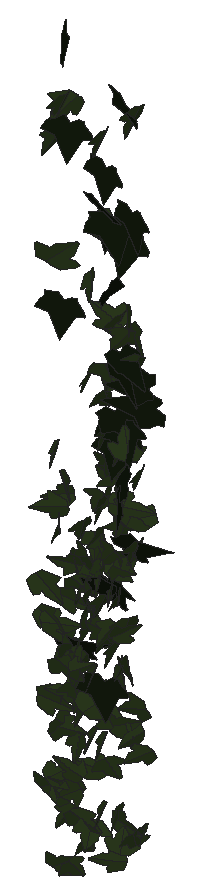
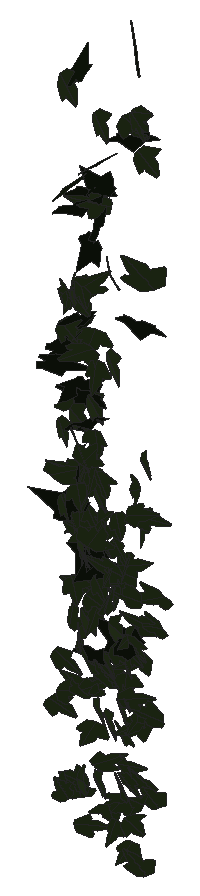
# SketchUp Ruby script. Lengths in inches.
U = 1.inch
M = Sketchup.active_model
def pt(a) = Geom::Point3d.new(a.map { |v| v * U })
def face(e, loops, mat)
  f = e.add_face(loops[0].map { |a| pt(a) })
  loops[1..].each { |l| e.add_face(l.map { |a| pt(a) }).erase! }
  f.material = f.back_material = mat if mat
  f
end
# faces: each face lists its corners as indices into pts; further lists are holes
def faces(e, pts, list, mat = nil) = list.each { |f| face(e, (f[0].is_a?(Array) ? f : [f]).map { |l| l.map { |i| pts[i] } }, mat) }
# xy, xz, yz: faces in a plane at the given z, y or x. An outline is a flat list of corners, or four numbers for a rectangle; further outlines are holes
def ring(l) = l.size == 4 ? [[l[0], l[1]], [l[2], l[1]], [l[2], l[3]], [l[0], l[3]]] : l.each_slice(2).to_a
def flat(e, list, mat, &to3) = list.each { |f| face(e, (f[0].is_a?(Array) ? f : [f]).map { |l| ring(l).map { |u, v| to3.(u, v) } }, mat) }
def xy(e, z, list, mat = nil) = flat(e, list, mat) { |x, y| [x, y, z] }
def xz(e, y, list, mat = nil) = flat(e, list, mat) { |x, z| [x, y, z] }
def yz(e, x, list, mat = nil) = flat(e, list, mat) { |y, z| [x, y, z] }
def lines(e, pts, list) = list.each { |a, b| e.add_line(pt(pts[a]), pt(pts[b])) }
# prism: a flat outline (further loops are holes) pulled along v
def prism(e, loops, v, mat = nil)
  f = face(e, loops, mat); d = Geom::Vector3d.new(v.map { |x| x * U })
  f.pushpull(f.normal.samedirection?(d) ? d.length : -d.length)
end
def box(e, o, s, mat = nil) = prism(e, [[o, [o[0] + s[0], o[1], o[2]], [o[0] + s[0], o[1] + s[1], o[2]], [o[0], o[1] + s[1], o[2]]]], [0, 0, s[2]], mat)
def at(x, y, z, deg = 0) = Geom::Transformation.translation(pt([x, y, z])) * Geom::Transformation.rotation(ORIGIN, Z_AXIS, deg.degrees)
def axes(o, x, y, z) = Geom::Transformation.new([*x, 0, *y, 0, *z, 0, *pt(o).to_a, 1])
def part(name) = M.definitions.add(name)
# library, detail: a bought-in or finely detailed component or shape, given as its bounding box
def library(name, o, s) = part(name).tap { |d| box(d.entities, o, s) }
def detail(e, o, s) = box(e.add_group.entities, o, s)
def put(e, d, t, mat = nil) = e.add_instance(d, t).tap { |i| i.material = mat if mat }
def group(e, t, mat = nil) = e.add_group.tap { |g| g.transformation = t; g.material = mat if mat }.entities
root = M.entities
M.materials.add("1026 AP 7946 SUNNY SIDE UP").color = [254, 231, 186]
M.materials.add("efeu1").color = [18, 25, 13]
M.materials.add("efeu2").color = [43, 57, 29]
c1 = part("ivyleaf_10")
p = [[0,0.5,-0.03],[-0.0625,2.02,-0.43],[-0.19,2.01,-0.46],[-0.54,1.05,-0.29],[-0.52,0.625,-0.18],[-0.83,0.76,-0.28],
  [-1.16,0.64,-0.33],[-1.15,0.33,-0.24],[-0.77,-0.39,0.02],[-0.3,-0.51,0.16],[0.04,-0.48,0.23],[-0.02,2.01,-0.4375],
  [-0.06,2.01,-0.43],[0.04,-0.49,0.23],[0.67,-0.49,0.14],[1.38,0.36,-0.2],[1.375,0.51,-0.24],[0.81,0.65,-0.19],
  [0.62,0.59,-0.15],[0.6,1.09,-0.28],[0.5,1.23,-0.31]]
faces(c1.entities,p,[[0,1,2,3,4,5,6,7,8,9,10],[11,12,0,13,14,15,16,17,18,19,20]],"efeu2")
c2 = part("ivyleaf_9")
p = [[1.54,2.16,1.25],[1.36,2.04,1.19],[-0.21,0.99,0.68],[-0.71,1.11,0.82],[-0.85,0.86,0.67],[-0.8,0.17,0.21],
  [-0.9,-0.01,0.1],[-0.67,-0.16,-0.02],[-0.08,-0.08,-0.05],[-0.03,-0.6,-0.4],[0.65,-0.88,-0.66],[0.83,-0.6,-0.49],
  [1.29,-0.42,-0.43],[1.8125,-0.07,-0.26],[1.21,0.44,0.15]]
faces(c2.entities,p,[[0,1,2,3,4,5,6,7,8,9,10,11,12,13,14]],"efeu1")
put(root,c1,axes([102.42,212.2,265.33],[-0.05183,-0.21859,0.1221],[-0.02891,-0.11834,-0.22843],[0.39086,-0.03774,-0.00071]),"1026 AP 7946 SUNNY SIDE UP")
put(root,c1,axes([102.56,212.09,256.98],[-0.05923,0.00088,0.22172],[-0.21902,-0.16665,-0.02539],[0.25797,-0.14129,0.02935]),"1026 AP 7946 SUNNY SIDE UP")
put(root,c1,axes([102.23,212.03,250.57],[-0.23389,-0.00224,0.14605],[0.22173,0.01927,0.15284],[-0.02344,0.20459,-0.01159]),"1026 AP 7946 SUNNY SIDE UP")
put(root,c1,axes([102.56,212.34,257.16],[0.04395,0.01091,-0.21592],[-0.2358,-0.14698,-0.02934],[-0.23101,0.1521,-0.01113]),"1026 AP 7946 SUNNY SIDE UP")
put(root,c1,axes([102.17,211.97,255.25],[0.2333,0.0549,0.18943],[0.28714,0.02973,-0.16105],[-0.09116,0.23415,-0.0225]),"1026 AP 7946 SUNNY SIDE UP")
put(root,c1,axes([102.32,212.16,262.48],[-0.3086,-0.12765,0.16703],[0.18784,0.11338,0.24052],[-0.26566,0.22845,-0.02396]),"1026 AP 7946 SUNNY SIDE UP")
put(root,c1,axes([102.18,212.08,252.53],[-0.01331,0.02689,0.24598],[0.37043,0.04719,0.0034],[-0.07315,0.23406,-0.02751]),"1026 AP 7946 SUNNY SIDE UP")
put(root,c1,axes([102.41,212.15,258.29],[0.1541,-0.14918,0.13102],[0.1011,-0.11086,-0.18444],[0.29211,0.11707,-0.00529]),"1026 AP 7946 SUNNY SIDE UP")
put(root,c1,axes([102.24,211.94,254.52],[0.14569,0.02064,0.19826],[0.30337,0.00552,-0.09633],[-0.02194,0.21341,-0.01542]),"1026 AP 7946 SUNNY SIDE UP")
put(root,c1,axes([102.58,212.17,266.1875],[-0.01205,-0.25163,0.02038],[0.00002,-0.02122,-0.25947],[0.39706,-0.00763,0.00063]),"1026 AP 7946 SUNNY SIDE UP")
put(root,c1,axes([102.66,212.34,266.1],[-0.17225,-0.16616,0.1834],[-0.04691,-0.18557,-0.1974],[0.38112,-0.09794,0.05859]),"1026 AP 7946 SUNNY SIDE UP")
put(root,c2,axes([102.52,212.25,261.53],[-0.27965,-0.12951,-0.11897],[0.17605,0.03932,-0.22426],[0.20743,-0.20797,0.02996]),"1026 AP 7946 SUNNY SIDE UP")
put(root,c1,axes([102.41,212.03,250.86],[0.24265,-0.05914,-0.13342],[0.21223,0.00149,0.16541],[-0.06973,-0.20124,0.03916]),"1026 AP 7946 SUNNY SIDE UP")
put(root,c1,axes([102.56,212.04,250.42],[0.08063,0.10781,-0.16909],[0.0979,0.15262,0.12375],[0.29369,-0.08048,0.00517]),"1026 AP 7946 SUNNY SIDE UP")
put(root,c1,axes([102.68,212.3,250.08],[-0.07739,-0.15273,0.1396],[-0.02077,-0.1376,-0.16447],[0.32129,-0.04568,0.023]),"1026 AP 7946 SUNNY SIDE UP")
put(root,c1,axes([102.82,212.22,252.8],[0.01424,0.05128,0.21413],[-0.18625,-0.17175,0.04804],[0.27989,-0.1169,0.02107]),"1026 AP 7946 SUNNY SIDE UP")
put(root,c1,axes([102.7,211.85,256.72],[0.06745,-0.18648,-0.15225],[-0.0089,0.14827,-0.19495],[0.373,0.03726,0.02288]),"1026 AP 7946 SUNNY SIDE UP")
put(root,c2,axes([102.57,212.17,267.3],[0.01695,0.10486,0.29048],[-0.0312,-0.28069,0.10691],[0.47113,-0.02236,-0.00337]),"1026 AP 7946 SUNNY SIDE UP")
put(root,c1,axes([102.58,212.01,248.9],[-0.24354,-0.04898,0.13473],[0.1849,0.06038,0.16676],[-0.11921,0.1937,-0.0166]),"1026 AP 7946 SUNNY SIDE UP")
put(root,c1,axes([102.92,212.125,255.79],[-0.06837,-0.00814,-0.20351],[-0.28154,-0.08405,0.04369],[-0.13167,0.18394,0.01225]),"1026 AP 7946 SUNNY SIDE UP")
put(root,c1,axes([102.62,212.14,257.65],[-0.12692,0.13096,-0.17686],[0.11265,-0.15749,-0.15871],[-0.32127,-0.10696,0.01422]),"1026 AP 7946 SUNNY SIDE UP")
put(root,c1,axes([102.6875,211.88,252.3],[-0.07438,-0.1403,-0.16599],[0.12276,0.14139,-0.15037],[0.31169,-0.08917,0.01961]),"1026 AP 7946 SUNNY SIDE UP")
put(root,c1,axes([102.46,211.89,254.41],[0.10281,-0.0584,-0.2315],[0.36069,-0.01766,0.07349],[-0.05309,-0.23305,0.05099]),"1026 AP 7946 SUNNY SIDE UP")
put(root,c1,axes([102.98,211.96,253.71],[0.04266,-0.03133,-0.2044],[-0.22189,0.13925,-0.04176],[0.22438,0.14367,-0.00243]),"1026 AP 7946 SUNNY SIDE UP")
put(root,c2,axes([102.75,212.17,265.66],[-0.19675,-0.21444,-0.05392],[0.06078,0.03653,-0.25511],[0.34127,-0.13014,0.01435]),"1026 AP 7946 SUNNY SIDE UP")
put(root,c1,axes([102.68,211.92,252.14],[-0.09751,-0.08449,-0.22089],[0.25031,0.14418,-0.10536],[0.26107,-0.16979,0.01851]),"1026 AP 7946 SUNNY SIDE UP")
put(root,c1,axes([103.04,212.04,251.13],[0.13519,0.04911,0.18644],[-0.28645,-0.02405,0.09589],[0.0681,-0.19866,0.03323]),"1026 AP 7946 SUNNY SIDE UP")
put(root,c1,axes([102.92,212.01,254.03],[0.29732,-0.07854,-0.09029],[-0.13811,0.01495,-0.21],[0.12238,0.20769,-0.01763]),"1026 AP 7946 SUNNY SIDE UP")
put(root,c1,axes([102.86,212.16,255.92],[-0.14583,0.19318,0.01576],[-0.02935,0.00675,-0.22025],[-0.30315,-0.09358,0.01375]),"1026 AP 7946 SUNNY SIDE UP")
put(root,c1,axes([103.06,211.96,250.81],[0.20798,-0.10881,-0.13206],[-0.17417,0.06528,-0.17529],[0.19792,0.17178,-0.01548]),"1026 AP 7946 SUNNY SIDE UP")
put(root,c1,axes([102.89,211.86,254.12],[-0.04918,-0.09837,-0.2139],[0.11689,0.19334,-0.10506],[0.34099,-0.08047,0.00517]),"1026 AP 7946 SUNNY SIDE UP")
put(root,c1,axes([102.79,211.88,253.63],[-0.27673,-0.04366,-0.16647],[0.25569,0.00951,-0.18532],[0.06083,-0.23857,0.02163]),"1026 AP 7946 SUNNY SIDE UP")
put(root,c1,axes([103.06,212.05,252.84],[0.09376,-0.12325,-0.15523],[-0.12344,0.12819,-0.13992],[0.27917,0.09807,-0.00973]),"1026 AP 7946 SUNNY SIDE UP")
put(root,c1,axes([102.98,212.03,253.12],[-0.17086,-0.17352,-0.04386],[0.05286,0.02792,-0.2103],[0.27554,-0.11295,0.01314]),"1026 AP 7946 SUNNY SIDE UP")
put(root,c1,axes([102.8125,212.3,250.6875],[0.04274,-0.07842,-0.2017],[0.16362,-0.1662,0.08268],[-0.28771,-0.10617,0.01706]),"1026 AP 7946 SUNNY SIDE UP")
put(root,c1,axes([103.23,212.07,256.1],[-0.16152,0.04977,0.17504],[-0.25782,0.04649,-0.11607],[-0.10388,-0.19278,0.01592]),"1026 AP 7946 SUNNY SIDE UP")
put(root,c1,axes([102.77,212.02,255.03],[0.00528,0.00675,0.22856],[0.33909,0.05229,-0.0047],[-0.0824,0.2156,-0.00468]),"1026 AP 7946 SUNNY SIDE UP")
put(root,c1,axes([103.1,212.06,252.5],[0.12326,-0.20103,-0.04777],[-0.03877,0.0389,-0.22188],[0.32167,0.08172,-0.00844]),"1026 AP 7946 SUNNY SIDE UP")
put(root,c1,axes([103.11,212.14,256.78],[-0.05662,-0.20051,-0.00689],[0.0054,0.00502,-0.20983],[0.31536,-0.03609,0.00236]),"1026 AP 7946 SUNNY SIDE UP")
put(root,c1,axes([103.13,212.14,253.77],[-0.04915,-0.16013,0.15046],[-0.01653,-0.14719,-0.16838],[0.34136,-0.03018,0.01351]),"1026 AP 7946 SUNNY SIDE UP")
put(root,c1,axes([103.04,211.84,249.1875],[-0.11377,-0.1537,-0.12737],[0.12053,0.09843,-0.17293],[0.28486,-0.10304,0.0223]),"1026 AP 7946 SUNNY SIDE UP")
put(root,c1,axes([102.88,212.08,253.43],[-0.04139,0.04846,0.24284],[0.32159,-0.11994,0.04829],[0.19861,0.20431,-0.02757]),"1026 AP 7946 SUNNY SIDE UP")
put(root,c1,axes([103.18,211.89,255.23],[0.11128,-0.07881,0.17769],[-0.13284,0.15225,0.10799],[-0.26767,-0.10832,0.02028]),"1026 AP 7946 SUNNY SIDE UP")
put(root,c1,axes([103.04,212.06,251.91],[0.26773,-0.10341,0.0825],[0.09244,-0.058,-0.20475],[0.18435,0.17926,-0.01715]),"1026 AP 7946 SUNNY SIDE UP")
put(root,c2,axes([102.86,212.03,253.94],[0.30809,0.10271,-0.10356],[0.11898,0.07193,0.22675],[0.19288,-0.20843,0.02556]),"1026 AP 7946 SUNNY SIDE UP")
put(root,c1,axes([103.04,212.03,255.52],[-0.22467,-0.07151,-0.12918],[0.18825,0.03883,-0.16366],[0.1258,-0.18582,0.01421]),"1026 AP 7946 SUNNY SIDE UP")
put(root,c1,axes([103.16,212.22,254.35],[0.07407,-0.16219,0.13708],[0.03445,-0.13277,-0.17429],[0.329,0.05042,-0.01261]),"1026 AP 7946 SUNNY SIDE UP")
put(root,c1,axes([103.38,212.33,251.19],[0.07303,0.11884,0.19021],[-0.14463,-0.16008,0.12952],[0.31253,-0.10185,0.01549]),"1026 AP 7946 SUNNY SIDE UP")
put(root,c1,axes([103.16,211.79,253.64],[0.00959,-0.00139,-0.20858],[0.15862,0.17564,0.00291],[0.27602,-0.10088,0.00557]),"1026 AP 7946 SUNNY SIDE UP")
put(root,c1,axes([103.08,211.97,250.24],[-0.21738,-0.03336,-0.16856],[0.25746,0.01335,-0.14542],[0.05003,-0.21364,0.01595]),"1026 AP 7946 SUNNY SIDE UP")
put(root,c1,axes([103.34,211.86,254.79],[0.0164,0.00633,0.20883],[-0.1605,0.17551,0.00079],[-0.27549,-0.10188,0.01197]),"1026 AP 7946 SUNNY SIDE UP")
put(root,c1,axes([103.26,212.03,249.68],[-0.04876,-0.16398,-0.13783],[0.05791,0.12803,-0.17088],[0.32676,-0.04716,0.00972]),"1026 AP 7946 SUNNY SIDE UP")
put(root,c1,axes([103.34,212.07,260.31],[0.09643,-0.24813,-0.00582],[-0.01578,0.00189,-0.26313],[0.38991,0.06144,-0.00921]),"1026 AP 7946 SUNNY SIDE UP")
put(root,c1,axes([103.33,212.17,254.73],[-0.19861,0.18378,0.04266],[0.03978,-0.0316,0.22953],[0.29318,0.12878,-0.00224]),"1026 AP 7946 SUNNY SIDE UP")
put(root,c1,axes([103.32,211.99,255.41],[0.00726,-0.06235,-0.22372],[0.03769,0.21577,-0.06214],[0.35273,-0.02177,0.01124]),"1026 AP 7946 SUNNY SIDE UP")
put(root,c1,axes([103.29,212.24,253.47],[0.17009,-0.17803,0.08565],[0.05265,-0.07799,-0.21476],[0.30513,0.1127,-0.01069]),"1026 AP 7946 SUNNY SIDE UP")
put(root,c1,axes([103.21,212.21,262.36],[0.18806,-0.08786,0.1941],[0.20585,-0.13776,-0.15219],[0.25485,0.17611,-0.02031]),"1026 AP 7946 SUNNY SIDE UP")
put(root,c1,axes([103.375,212.11,252.11],[0.14124,-0.20103,0.02572],[0.00401,-0.02743,-0.22681],[0.31873,0.08943,-0.00854]),"1026 AP 7946 SUNNY SIDE UP")
put(root,c1,axes([103.37,212.0625,250.07],[0.25201,0.1629,-0.05602],[-0.04341,-0.05025,-0.2352],[-0.26699,0.16193,-0.01464]),"1026 AP 7946 SUNNY SIDE UP")
put(root,c1,axes([103.15,212.2,255.57],[0.03754,-0.02577,-0.25044],[0.36136,-0.08047,0.03159],[-0.13037,-0.23048,0.01544]),"1026 AP 7946 SUNNY SIDE UP")
put(root,c1,axes([103.36,212.17,256.53],[0.2866,-0.05607,0.07568],[0.10178,-0.03947,-0.19586],[0.10427,0.19263,-0.01684]),"1026 AP 7946 SUNNY SIDE UP")
put(root,c1,axes([103.3,212.13,252.97],[0.27312,-0.10567,-0.10763],[0.16245,-0.02837,0.20753],[-0.16702,-0.20039,0.02585]),"1026 AP 7946 SUNNY SIDE UP")
put(root,c1,axes([103.5,212.27,257.28],[0.08399,-0.19633,0.04337],[0.01385,-0.04238,-0.20984],[0.31579,0.05407,-0.00233]),"1026 AP 7946 SUNNY SIDE UP")
put(root,c1,axes([103.63,212.13,257.56],[-0.29341,-0.03001,0.08155],[-0.1136,-0.04421,-0.19255],[0.06988,-0.19789,0.02941]),"1026 AP 7946 SUNNY SIDE UP")
put(root,c1,axes([103.52,212.09,254.5625],[-0.08816,0.14621,0.17135],[0.06794,-0.16018,0.15993],[0.34052,0.06981,0.01246]),"1026 AP 7946 SUNNY SIDE UP")
put(root,c1,axes([103.54,212.16,256.625],[0.02416,0.02793,-0.22301],[-0.06169,-0.21329,-0.03245],[-0.33787,0.04094,-0.01002]),"1026 AP 7946 SUNNY SIDE UP")
put(root,c1,axes([103.58,212.19,255.22],[-0.02723,-0.21131,0.04356],[-0.00134,-0.04355,-0.21866],[0.33923,-0.01714,0.00263]),"1026 AP 7946 SUNNY SIDE UP")
put(root,c1,axes([103.69,212.25,256.11],[-0.30435,-0.08019,-0.10827],[-0.15876,-0.02934,0.2154],[-0.13328,0.21806,-0.00936]),"1026 AP 7946 SUNNY SIDE UP")
put(root,c1,axes([103.6,212.14,265.74],[0.0393,-0.24742,0.0431],[0.00535,-0.04312,-0.25644],[0.3949,0.02521,-0.00081]),"1026 AP 7946 SUNNY SIDE UP")
put(root,c2,axes([103.5,212.36,264.83],[-0.05906,-0.24353,0.07287],[0.00537,-0.07337,-0.25387],[0.39932,-0.03503,0.01419]),"1026 AP 7946 SUNNY SIDE UP")
put(root,c2,axes([103.42,212.34,263.42],[0.15758,-0.08231,-0.22732],[0.29506,-0.11615,0.13204],[-0.22262,-0.21221,0.0141]),"1026 AP 7946 SUNNY SIDE UP")
put(root,c1,axes([103.77,212.0625,258.41],[-0.2881,0.06721,0.07861],[-0.12161,0.00878,-0.20022],[-0.10311,-0.19814,0.0165]),"1026 AP 7946 SUNNY SIDE UP")
put(root,c2,axes([103.49,212.01,255.625],[0.38935,0.03743,0.01849],[0.03271,-0.01945,-0.25708],[-0.05632,0.24749,-0.02151]),"1026 AP 7946 SUNNY SIDE UP")
put(root,c1,axes([103.7,212.09,257.62],[-0.03665,-0.15707,-0.15809],[0.03322,0.1511,-0.1627],[0.3427,-0.03145,-0.00113]),"1026 AP 7946 SUNNY SIDE UP")
put(root,c1,axes([103.81,212.29,257.97],[-0.17098,-0.12097,-0.17067],[-0.18148,-0.11799,0.1668],[-0.2656,0.1585,-0.0041]),"1026 AP 7946 SUNNY SIDE UP")
put(root,c1,axes([103.6875,212.11,254.4],[-0.0316,-0.16282,-0.16751],[0.05357,0.15838,-0.16775],[0.35679,-0.0382,0.01035]),"1026 AP 7946 SUNNY SIDE UP")
put(root,c1,axes([103.68,212.0625,250.58],[0.14779,-0.18701,0.06797],[0.02997,-0.06534,-0.21566],[0.31094,0.09518,-0.01152]),"1026 AP 7946 SUNNY SIDE UP")
put(root,c1,axes([103.71,212.0625,259.99],[-0.06914,-0.22823,-0.13197],[0.03553,0.12478,-0.23871],[0.409,-0.04942,-0.00157]),"1026 AP 7946 SUNNY SIDE UP")
put(root,c1,axes([103.51,211.8125,252.89],[0.2344,0.07573,-0.19117],[0.24342,0.10421,0.17214],[0.20114,-0.21437,0.01445]),"1026 AP 7946 SUNNY SIDE UP")
put(root,c1,axes([103.61,212.02,256.05],[0.22754,-0.13212,0.1317],[0.13606,-0.09567,-0.20215],[0.25599,0.16829,-0.00962]),"1026 AP 7946 SUNNY SIDE UP")
put(root,c1,axes([103.7,212.04,252.1875],[0.17133,-0.16213,0.09371],[0.06251,-0.08377,-0.20132],[0.28628,0.11532,-0.01212]),"1026 AP 7946 SUNNY SIDE UP")
put(root,c2,axes([103.51,212.12,264.0625],[0.05427,-0.11716,0.22293],[0.19172,-0.18242,-0.12248],[0.33715,0.12259,0.03376]),"1026 AP 7946 SUNNY SIDE UP")
put(root,c1,axes([103.79,212.1,259.19],[0.06589,-0.23974,0.07743],[0.01347,-0.07617,-0.25113],[0.39548,0.04254,-0.00435]),"1026 AP 7946 SUNNY SIDE UP")
put(root,c1,axes([103.9,212.07,252.6],[0.07918,0.11123,0.17109],[-0.12298,-0.14593,0.12475],[0.28834,-0.09279,0.00623]),"1026 AP 7946 SUNNY SIDE UP")
put(root,c1,axes([103.84,212.1,254.71],[-0.07321,-0.13963,0.16171],[0.02852,-0.16363,-0.14464],[0.33005,-0.01683,0.04837]),"1026 AP 7946 SUNNY SIDE UP")
put(root,c2,axes([103.77,211.99,253.46],[-0.24645,-0.15918,-0.12093],[0.14889,0.06979,-0.22911],[0.27207,-0.18238,0.01584]),"1026 AP 7946 SUNNY SIDE UP")
put(root,c1,axes([103.78,212.29,257.19],[-0.06481,0.16581,-0.12461],[0.03623,-0.11982,-0.17663],[-0.32156,-0.04692,0.00521]),"1026 AP 7946 SUNNY SIDE UP")
put(root,c1,axes([104.02,212.125,249.46],[-0.02251,0.03872,0.2144],[-0.19351,-0.17097,0.02308],[0.2704,-0.11913,0.03436]),"1026 AP 7946 SUNNY SIDE UP")
put(root,c1,axes([104.04,211.92,256.51],[-0.24079,0.06768,0.12884],[-0.20625,0.00233,-0.16726],[-0.08497,-0.19746,0.04089]),"1026 AP 7946 SUNNY SIDE UP")
put(root,c1,axes([103.59,212.04,263.73],[0.08423,-0.03541,-0.26858],[0.39667,0.08176,0.04247],[0.11637,-0.25308,0.04963]),"1026 AP 7946 SUNNY SIDE UP")
put(root,c1,axes([103.85,211.98,251.7],[-0.19577,-0.1452,-0.10433],[0.12986,0.06074,-0.19555],[0.24538,-0.14799,0.02025]),"1026 AP 7946 SUNNY SIDE UP")
put(root,c1,axes([104.02,212.03,261.71],[0.13265,0.19018,0.16479],[-0.13112,-0.13626,0.21284],[0.36694,-0.11744,0.01649]),"1026 AP 7946 SUNNY SIDE UP")
put(root,c1,axes([103.89,211.95,260.63],[-0.29963,-0.10982,-0.05445],[0.09201,0.00231,-0.22492],[0.16763,-0.19757,0.02613]),"1026 AP 7946 SUNNY SIDE UP")
put(root,c1,axes([103.95,212.11,254.29],[0.04843,-0.21778,0.07231],[0.00503,-0.07165,-0.2269],[0.36034,0.03027,-0.00655]),"1026 AP 7946 SUNNY SIDE UP")
put(root,c2,axes([103.9,212.27,258.76],[-0.14717,-0.22721,0.01375],[0.00154,-0.01622,-0.25314],[0.35801,-0.09333,0.00674]),"1026 AP 7946 SUNNY SIDE UP")
put(root,c1,axes([103.9375,212.25,255.8],[0.20688,-0.18877,0.04926],[0.02016,-0.05048,-0.23662],[0.30596,0.13097,-0.01772]),"1026 AP 7946 SUNNY SIDE UP")
put(root,c2,axes([103.89,211.99,255.79],[0.36756,0.00677,-0.10213],[-0.15395,-0.02817,-0.23988],[-0.02704,0.25236,-0.02254]),"1026 AP 7946 SUNNY SIDE UP")
put(root,c1,axes([103.875,212.07,255.75],[0.17083,-0.14536,0.14307],[0.13692,-0.1093,-0.18756],[0.28592,0.13919,0.00434]),"1026 AP 7946 SUNNY SIDE UP")
put(root,c1,axes([103.96,212.18,257.71],[-0.16177,0.17725,-0.03853],[0.01414,-0.03912,-0.21102],[-0.28483,-0.10261,0.01141]),"1026 AP 7946 SUNNY SIDE UP")
put(root,c2,axes([104.07,211.76,262.57],[-0.06438,0.0362,-0.25803],[-0.22229,0.20743,0.05586],[0.33045,0.14659,-0.0127]),"1026 AP 7946 SUNNY SIDE UP")
put(root,c1,axes([103.86,212.33,253.66],[0.13355,-0.0719,0.1761],[0.22514,-0.09476,-0.11463],[0.18624,0.16612,0.0123]),"1026 AP 7946 SUNNY SIDE UP")
put(root,c1,axes([103.97,212.23,250.55],[0.08896,-0.11105,0.18407],[0.11264,-0.16449,-0.1292],[0.31193,0.09107,-0.00584]),"1026 AP 7946 SUNNY SIDE UP")
put(root,c2,axes([103.93,212,263.94],[-0.14767,-0.23279,-0.1053],[0.07959,0.08823,-0.25774],[0.39093,-0.1059,0.0127]),"1026 AP 7946 SUNNY SIDE UP")
put(root,c1,axes([104.08,212.08,261.79],[-0.02986,-0.2424,-0.01632],[-0.00108,0.01456,-0.25039],[0.38182,-0.01892,-0.00198]),"1026 AP 7946 SUNNY SIDE UP")
put(root,c1,axes([104.1,212.1,253.9],[0.05013,-0.16369,-0.12664],[-0.0275,0.12084,-0.17102],[0.31983,0.03605,0.00514]),"1026 AP 7946 SUNNY SIDE UP")
put(root,c1,axes([104.11,212.15,257.09],[-0.17991,-0.174,0.01432],[0.00203,-0.01864,-0.21433],[0.27459,-0.11387,0.01096]),"1026 AP 7946 SUNNY SIDE UP")
put(root,c1,axes([103.9,212.16,260.34],[-0.17243,-0.0929,-0.18639],[0.28329,0.04977,-0.13893],[0.14679,-0.20516,0.04918]),"1026 AP 7946 SUNNY SIDE UP")
put(root,c2,axes([104.32,211.99,258.16],[-0.07748,-0.01067,-0.26156],[-0.37323,0.09413,0.04394],[0.14245,0.24083,-0.02714]),"1026 AP 7946 SUNNY SIDE UP")
put(root,c1,axes([104.14,212.21,258.86],[0.03845,-0.19162,0.11578],[0.00782,-0.11366,-0.19949],[0.35008,0.02358,-0.00826]),"1026 AP 7946 SUNNY SIDE UP")
put(root,c1,axes([103.93,212.03,256.05],[0.22546,0.03985,-0.18028],[0.24336,0.08652,0.15125],[0.14358,-0.20923,0.02673]),"1026 AP 7946 SUNNY SIDE UP")
put(root,c2,axes([103.99,212.1,259.59],[0.00396,-0.18754,-0.19322],[0.02968,0.18615,-0.1915],[0.41481,-0.01153,0.01555]),"1026 AP 7946 SUNNY SIDE UP")
put(root,c1,axes([104.18,211.88,255.6],[0.01713,-0.18213,-0.12164],[-0.01267,0.11677,-0.18728],[0.34018,0.01352,-0.00085]),"1026 AP 7946 SUNNY SIDE UP")
put(root,c1,axes([104.25,212.11,261.47],[-0.19304,-0.15313,0.11924],[-0.08946,-0.10326,-0.202],[0.28913,-0.13419,0.01711]),"1026 AP 7946 SUNNY SIDE UP")
put(root,c1,axes([103.98,212.04,252.52],[-0.2188,-0.03779,0.18764],[0.25709,0.08419,0.147],[-0.14019,0.21338,-0.02329]),"1026 AP 7946 SUNNY SIDE UP")
put(root,c1,axes([104.23,212.15,254.94],[-0.118,-0.2084,0.00967],[0.00496,-0.01237,-0.22814],[0.32806,-0.07477,0.00693]),"1026 AP 7946 SUNNY SIDE UP")
put(root,c2,axes([104.09,212.22,266.55],[0.25671,-0.19301,-0.10963],[0.12146,-0.07247,0.25975],[-0.32369,-0.18026,0.01053]),"1026 AP 7946 SUNNY SIDE UP")
put(root,c2,axes([104.08,212.1,259.33],[-0.22325,-0.138,-0.17127],[0.22195,0.09014,-0.2017],[0.25596,-0.19852,0.02552]),"1026 AP 7946 SUNNY SIDE UP")
put(root,c2,axes([104.08,212.125,257.71],[0.00088,-0.01539,-0.26702],[0.32187,-0.15928,0.00928],[-0.25094,-0.20436,0.01096]),"1026 AP 7946 SUNNY SIDE UP")
put(root,c2,axes([104.1875,212.21,263.59],[-0.17686,-0.25437,0.01399],[0.00456,-0.0177,-0.28645],[0.40064,-0.11209,0.00943]),"1026 AP 7946 SUNNY SIDE UP")
put(root,c1,axes([104.09,212.35,261.7],[0.02392,-0.02834,0.26349],[0.2592,-0.19587,-0.03359],[0.31103,0.16542,0.00772]),"1026 AP 7946 SUNNY SIDE UP")
put(root,c1,axes([104.1,212.26,256.36],[-0.13222,0.07147,0.19635],[0.26463,-0.09082,0.11128],[0.17898,0.18707,-0.01948]),"1026 AP 7946 SUNNY SIDE UP")
put(root,c1,axes([104.33,212.29,260.82],[-0.05922,-0.19965,0.1183],[-0.02242,-0.11527,-0.20988],[0.36236,-0.03976,0.00635]),"1026 AP 7946 SUNNY SIDE UP")
put(root,c1,axes([104.1875,211.86,256.29],[-0.06648,-0.11618,-0.17473],[0.16306,0.1367,-0.12278],[0.27813,-0.10791,0.03022]),"1026 AP 7946 SUNNY SIDE UP")
put(root,c2,axes([104.16,212.06,260.99],[0.05204,-0.1956,-0.17619],[-0.04487,0.1675,-0.20339],[0.40492,0.0437,0.00011]),"1026 AP 7946 SUNNY SIDE UP")
put(root,c1,axes([104.32,212.31,266.43],[0.01893,-0.27357,0.09269],[0.02353,-0.09089,-0.28243],[0.45299,0.01615,0.0108]),"1026 AP 7946 SUNNY SIDE UP")
put(root,c2,axes([104.11,212.02,260.72],[0.1405,-0.25079,0.03625],[0.0066,-0.03735,-0.27435],[0.39847,0.08905,-0.00824]),"1026 AP 7946 SUNNY SIDE UP")
put(root,c1,axes([104.05,212.07,250.4],[0.01992,-0.01199,0.22739],[0.34752,-0.00631,-0.01345],[0.011,0.22107,0.01324]),"1026 AP 7946 SUNNY SIDE UP")
put(root,c2,axes([104.18,212.34,264.05],[0.02902,-0.26189,0.07948],[0.00572,-0.07858,-0.27092],[0.42992,0.01872,-0.00176]),"1026 AP 7946 SUNNY SIDE UP")
put(root,c1,axes([104.22,211.86,254.73],[-0.05756,-0.12293,0.17051],[0.09444,0.15519,0.13278],[-0.31105,0.06987,0.00876]),"1026 AP 7946 SUNNY SIDE UP")
put(root,c1,axes([104.29,211.85,249.96],[0.22909,0.13662,-0.0556],[0.04421,0.04978,0.20535],[0.22717,-0.14746,0.0161]),"1026 AP 7946 SUNNY SIDE UP")
put(root,c1,axes([104.03,212.11,257.53],[0.02421,-0.06621,-0.25776],[0.40636,0.00716,0.0145],[0.00522,-0.2502,0.06705]),"1026 AP 7946 SUNNY SIDE UP")
put(root,c2,axes([104.54,212.34,260.23],[-0.1405,-0.03911,0.22931],[-0.29473,-0.12133,-0.10009],[0.19916,-0.20714,0.01366]),"1026 AP 7946 SUNNY SIDE UP")
put(root,c1,axes([104.37,211.95,258.875],[0.19796,0.22418,-0.04108],[0.01127,0.0431,0.2647],[0.35821,-0.12525,0.01438]),"1026 AP 7946 SUNNY SIDE UP")
put(root,c1,axes([104.62,212.1,253.12],[-0.14278,0.01083,0.19514],[-0.29699,-0.02427,-0.09202],[0.02714,-0.20859,0.0196]),"1026 AP 7946 SUNNY SIDE UP")
put(root,c1,axes([104.58,212.19,257.3],[0.20527,0.12214,0.18664],[-0.25086,-0.08976,0.18093],[0.23343,-0.20386,0.03031]),"1026 AP 7946 SUNNY SIDE UP")
put(root,c1,axes([104.44,212.18,256.74],[-0.00099,-0.22509,0.03075],[-0.00014,-0.03113,-0.23207],[0.35729,-0.00064,-0.00001]),"1026 AP 7946 SUNNY SIDE UP")
put(root,c1,axes([104.43,212.21,252.43],[-0.04529,-0.05134,0.23084],[0.02235,-0.22608,-0.05274],[0.36122,0.00755,0.0322]),"1026 AP 7946 SUNNY SIDE UP")
put(root,c1,axes([104.43,211.93,253.9],[-0.27466,0.16166,0.03969],[0.0596,-0.01431,0.24461],[0.25409,0.1781,-0.01447]),"1026 AP 7946 SUNNY SIDE UP")
put(root,c1,axes([104.43,212.16,250.04],[-0.03059,-0.1913,0.06501],[0.006,0.06413,0.19845],[-0.31723,0.01966,-0.00251]),"1026 AP 7946 SUNNY SIDE UP")
put(root,c2,axes([104.76,212.3,259.87],[-0.13005,-0.13315,-0.21101],[-0.19978,-0.16032,0.15987],[-0.32693,0.15093,-0.01376]),"1026 AP 7946 SUNNY SIDE UP")
put(root,c1,axes([104.33,212.24,261.48],[-0.09474,0.09051,-0.241],[0.16646,-0.20952,-0.11258],[-0.3584,-0.12124,0.01142]),"1026 AP 7946 SUNNY SIDE UP")
put(root,c1,axes([104.66,212.21,252.09],[-0.1513,-0.07896,0.16705],[-0.15406,-0.13202,-0.12655],[0.23886,-0.13517,0.0242]),"1026 AP 7946 SUNNY SIDE UP")
put(root,c1,axes([104.55,212.14,258.43],[0.04416,-0.21069,0.00302],[0.00063,-0.00411,-0.219],[0.33136,0.02809,0.00001]),"1026 AP 7946 SUNNY SIDE UP")
put(root,c1,axes([104.54,211.95,250.29],[-0.08829,-0.19844,-0.08409],[0.03933,0.07657,-0.21199],[0.33442,-0.0614,0.00273]),"1026 AP 7946 SUNNY SIDE UP")
put(root,c2,axes([104.22,212.13,256.6],[0.11335,-0.02915,0.24086],[0.35948,-0.05115,-0.07943],[0.09061,0.23941,0.01384]),"1026 AP 7946 SUNNY SIDE UP")
